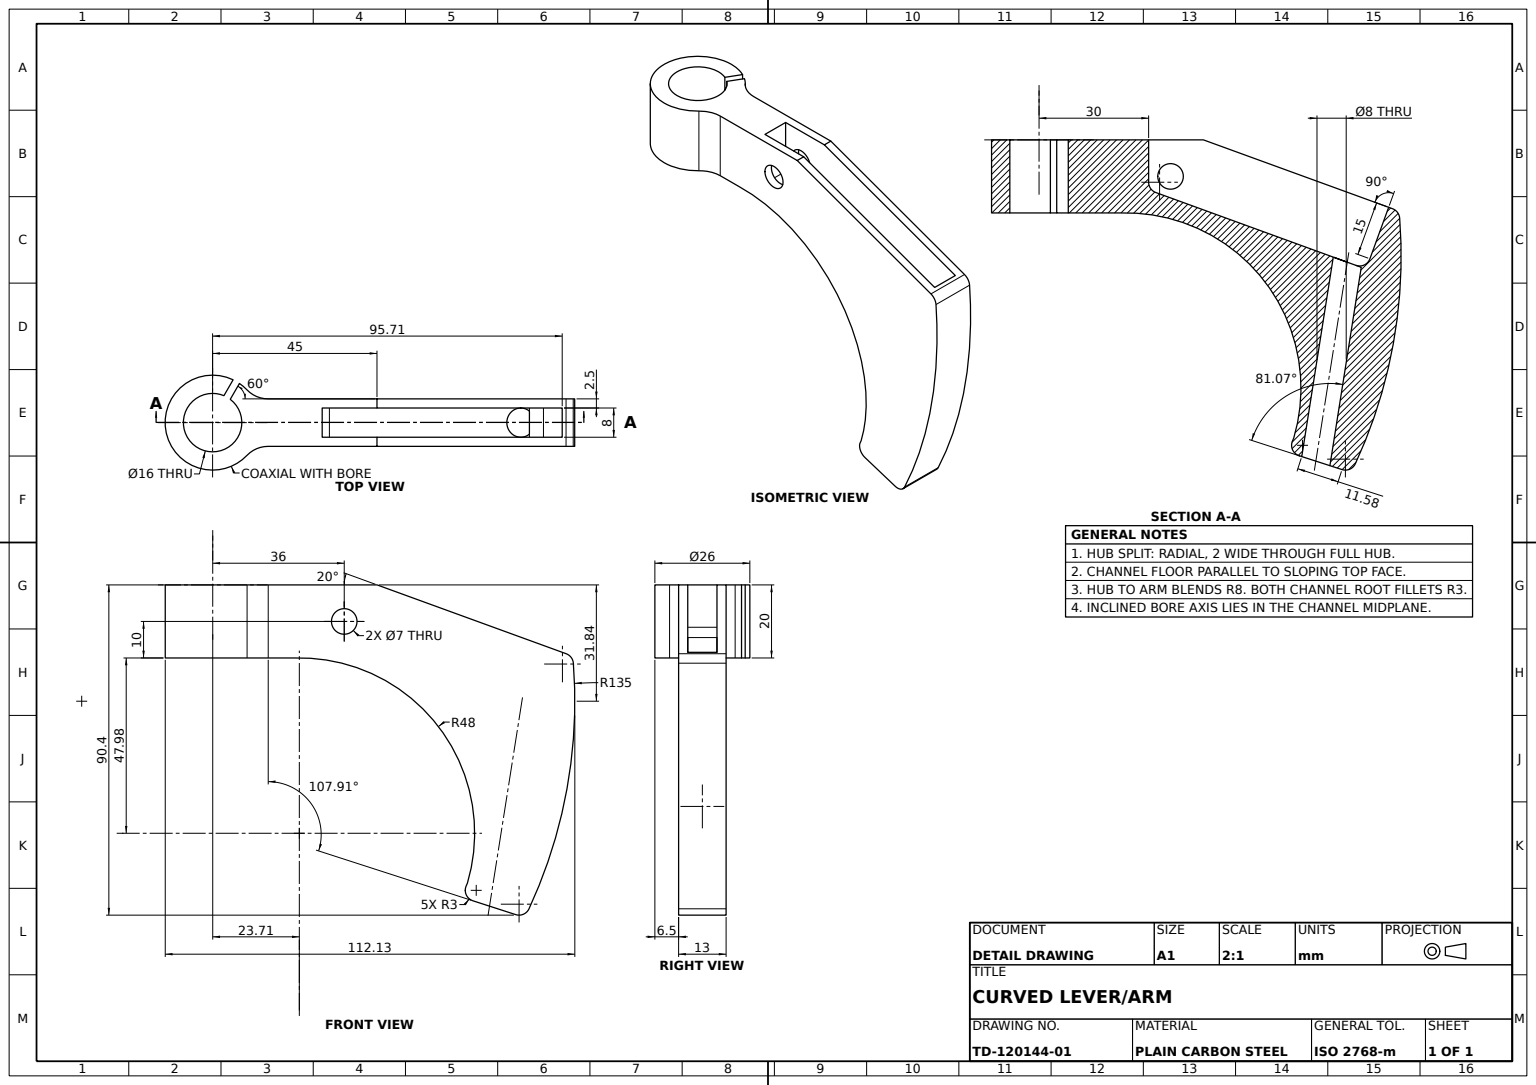
ISO-10303-21;
HEADER;
FILE_DESCRIPTION((''),'2;1');
FILE_NAME('','',(''),(''),'','','');
FILE_SCHEMA(('AUTOMOTIVE_DESIGN'));
ENDSEC;
DATA;
#1=APPLICATION_CONTEXT('');
#2=PRODUCT_CONTEXT('',#1,'mechanical');
#3=PRODUCT('','','',(#2));
#4=PRODUCT_DEFINITION_FORMATION('','',#3);
#5=PRODUCT_DEFINITION_CONTEXT('',#1,'design');
#6=PRODUCT_DEFINITION('','',#4,#5);
#7=PRODUCT_DEFINITION_SHAPE('','',#6);
#8=(LENGTH_UNIT()NAMED_UNIT(*)SI_UNIT(.MILLI.,.METRE.));
#9=(NAMED_UNIT(*)PLANE_ANGLE_UNIT()SI_UNIT($,.RADIAN.));
#10=(NAMED_UNIT(*)SI_UNIT($,.STERADIAN.)SOLID_ANGLE_UNIT());
#11=UNCERTAINTY_MEASURE_WITH_UNIT(LENGTH_MEASURE(1.E-05),#8,'distance_accuracy_value','');
#12=(GEOMETRIC_REPRESENTATION_CONTEXT(3)GLOBAL_UNCERTAINTY_ASSIGNED_CONTEXT((#11))GLOBAL_UNIT_ASSIGNED_CONTEXT((#8,#9,#10))REPRESENTATION_CONTEXT('',''));
#13=CARTESIAN_POINT('',(39.5,-10.,2.5));
#14=VERTEX_POINT('',#13);
#15=CARTESIAN_POINT('',(39.5,-10.,0.));
#16=VERTEX_POINT('',#15);
#17=CARTESIAN_POINT('',(39.5,-10.,13.));
#18=DIRECTION('',(0.,0.,-1.));
#19=VECTOR('',#18,1000.);
#20=LINE('',#17,#19);
#21=EDGE_CURVE('',#14,#16,#20,.T.);
#22=ORIENTED_EDGE('',*,*,#21,.F.);
#23=CARTESIAN_POINT('',(32.5,-10.,2.5));
#24=VERTEX_POINT('',#23);
#25=CARTESIAN_POINT('',(36.,-10.,2.5));
#26=DIRECTION('',(0.,0.,1.));
#27=DIRECTION('',(1.,0.,0.));
#28=AXIS2_PLACEMENT_3D('',#25,#26,#27);
#29=CIRCLE('',#28,3.5);
#30=EDGE_CURVE('',#14,#24,#29,.T.);
#31=ORIENTED_EDGE('',*,*,#30,.T.);
#32=CARTESIAN_POINT('',(32.5,-10.,0.));
#33=VERTEX_POINT('',#32);
#34=CARTESIAN_POINT('',(32.5,-10.,13.));
#35=LINE('',#34,#19);
#36=EDGE_CURVE('',#24,#33,#35,.T.);
#37=ORIENTED_EDGE('',*,*,#36,.T.);
#38=CARTESIAN_POINT('',(36.,-10.,0.));
#39=AXIS2_PLACEMENT_3D('',#38,#26,#27);
#40=CIRCLE('',#39,3.5);
#41=EDGE_CURVE('',#16,#33,#40,.T.);
#42=ORIENTED_EDGE('',*,*,#41,.F.);
#43=EDGE_LOOP('',(#22,#31,#37,#42));
#44=FACE_OUTER_BOUND('',#43,.T.);
#45=CARTESIAN_POINT('',(36.,-10.,13.));
#46=DIRECTION('',(-1.,0.,0.));
#47=AXIS2_PLACEMENT_3D('',#45,#18,#46);
#48=CYLINDRICAL_SURFACE('',#47,3.5);
#49=ADVANCED_FACE('',(#44),#48,.F.);
#50=CARTESIAN_POINT('',(30.,-11.595024,2.5));
#51=VERTEX_POINT('',#50);
#52=CARTESIAN_POINT('',(30.,-11.595024,10.5));
#53=VERTEX_POINT('',#52);
#54=VECTOR('',#26,1000.);
#55=LINE('',#50,#54);
#56=EDGE_CURVE('',#51,#53,#55,.T.);
#57=ORIENTED_EDGE('',*,*,#56,.T.);
#58=CARTESIAN_POINT('',(31.97394,-14.414102,10.5));
#59=VERTEX_POINT('',#58);
#60=CARTESIAN_POINT('',(33.,-11.595024,10.5));
#61=AXIS2_PLACEMENT_3D('',#60,#26,#46);
#62=CIRCLE('',#61,3.);
#63=EDGE_CURVE('',#53,#59,#62,.T.);
#64=ORIENTED_EDGE('',*,*,#63,.T.);
#65=CARTESIAN_POINT('',(31.97394,-14.414102,2.5));
#66=VERTEX_POINT('',#65);
#67=LINE('',#65,#54);
#68=EDGE_CURVE('',#66,#59,#67,.T.);
#69=ORIENTED_EDGE('',*,*,#68,.F.);
#70=CARTESIAN_POINT('',(33.,-11.595024,2.5));
#71=AXIS2_PLACEMENT_3D('',#70,#26,#46);
#72=CIRCLE('',#71,3.);
#73=EDGE_CURVE('',#51,#66,#72,.T.);
#74=ORIENTED_EDGE('',*,*,#73,.F.);
#75=EDGE_LOOP('',(#57,#64,#69,#74));
#76=FACE_OUTER_BOUND('',#75,.T.);
#77=AXIS2_PLACEMENT_3D('',#70,#26,#27);
#78=CYLINDRICAL_SURFACE('',#77,3.);
#79=ADVANCED_FACE('',(#76),#78,.F.);
#80=CARTESIAN_POINT('',(90.578301,-32.551811,10.5));
#81=VERTEX_POINT('',#80);
#82=CARTESIAN_POINT('',(95.708603,-18.456422,10.5));
#83=VERTEX_POINT('',#82);
#84=DIRECTION('',(0.342020143,0.939692621,0.));
#85=VECTOR('',#84,1000.);
#86=LINE('',#80,#85);
#87=EDGE_CURVE('',#81,#83,#86,.T.);
#88=ORIENTED_EDGE('',*,*,#87,.T.);
#89=CARTESIAN_POINT('',(95.708603,-18.456422,2.5));
#90=VERTEX_POINT('',#89);
#91=LINE('',#89,#54);
#92=EDGE_CURVE('',#90,#83,#91,.T.);
#93=ORIENTED_EDGE('',*,*,#92,.F.);
#94=CARTESIAN_POINT('',(90.578301,-32.551811,2.5));
#95=VERTEX_POINT('',#94);
#96=LINE('',#94,#85);
#97=EDGE_CURVE('',#95,#90,#96,.T.);
#98=ORIENTED_EDGE('',*,*,#97,.F.);
#99=LINE('',#94,#54);
#100=EDGE_CURVE('',#95,#81,#99,.T.);
#101=ORIENTED_EDGE('',*,*,#100,.T.);
#102=EDGE_LOOP('',(#88,#93,#98,#101));
#103=FACE_OUTER_BOUND('',#102,.T.);
#104=DIRECTION('',(0.939692621,-0.342020143,0.));
#105=AXIS2_PLACEMENT_3D('',#94,#104,#84);
#106=PLANE('',#105);
#107=ADVANCED_FACE('',(#103),#106,.F.);
#108=CARTESIAN_POINT('',(0.,-20.,-6.5));
#109=VERTEX_POINT('',#108);
#110=CARTESIAN_POINT('',(5.614715,-20.,-5.224972));
#111=VERTEX_POINT('',#110);
#112=CARTESIAN_POINT('',(0.,-20.,6.5));
#113=DIRECTION('',(0.,-1.,0.));
#114=AXIS2_PLACEMENT_3D('',#112,#113,#18);
#115=CIRCLE('',#114,13.);
#116=EDGE_CURVE('',#109,#111,#115,.T.);
#117=ORIENTED_EDGE('',*,*,#116,.F.);
#118=CARTESIAN_POINT('',(0.,0.,-6.5));
#119=VERTEX_POINT('',#118);
#120=VECTOR('',#113,1000.);
#121=LINE('',#108,#120);
#122=EDGE_CURVE('',#119,#109,#121,.T.);
#123=ORIENTED_EDGE('',*,*,#122,.F.);
#124=CARTESIAN_POINT('',(5.614715,0.,-5.224972));
#125=VERTEX_POINT('',#124);
#126=CARTESIAN_POINT('',(0.,0.,6.5));
#127=AXIS2_PLACEMENT_3D('',#126,#113,#18);
#128=CIRCLE('',#127,13.);
#129=EDGE_CURVE('',#119,#125,#128,.T.);
#130=ORIENTED_EDGE('',*,*,#129,.T.);
#131=LINE('',#110,#120);
#132=EDGE_CURVE('',#125,#111,#131,.T.);
#133=ORIENTED_EDGE('',*,*,#132,.T.);
#134=EDGE_LOOP('',(#117,#123,#130,#133));
#135=FACE_OUTER_BOUND('',#134,.T.);
#136=CYLINDRICAL_SURFACE('',#114,13.);
#137=ADVANCED_FACE('',(#135),#136,.T.);
#138=CARTESIAN_POINT('',(86.733162,-34.344829,9.653567));
#139=VERTEX_POINT('',#138);
#140=CARTESIAN_POINT('',(88.206809,-34.881192,6.5));
#141=VERTEX_POINT('',#140);
#142=CARTESIAN_POINT('',(87.680002,-34.68945,8.881841));
#143=CARTESIAN_POINT('',(88.206809,-34.881192,7.754486));
#144=(BOUNDED_CURVE()B_SPLINE_CURVE(3,(#138,#142,#143,#140),.UNSPECIFIED.,.F.,.T.)B_SPLINE_CURVE_WITH_KNOTS((4,4),(2.233402225,3.141592654),.UNSPECIFIED.)CURVE()GEOMETRIC_REPRESENTATION_ITEM()RATIONAL_B_SPLINE_CURVE((1.,0.932438853,0.932438853,1.))REPRESENTATION_ITEM(''));
#145=EDGE_CURVE('',#139,#141,#144,.T.);
#146=ORIENTED_EDGE('',*,*,#145,.T.);
#147=CARTESIAN_POINT('',(79.625923,-89.179734,6.5));
#148=VERTEX_POINT('',#147);
#149=CARTESIAN_POINT('',(78.754253,-94.695526,6.5));
#150=DIRECTION('',(0.156094482,0.987742129,0.));
#151=VECTOR('',#150,1000.);
#152=LINE('',#149,#151);
#153=EDGE_CURVE('',#148,#141,#152,.T.);
#154=ORIENTED_EDGE('',*,*,#153,.F.);
#155=CARTESIAN_POINT('',(71.920122,-86.689858,6.5));
#156=VERTEX_POINT('',#155);
#157=CARTESIAN_POINT('',(71.920122,-86.689858,14.5));
#158=CARTESIAN_POINT('',(79.625923,-89.179734,14.5));
#159=(BOUNDED_CURVE()B_SPLINE_CURVE(3,(#155,#157,#158,#147),.UNSPECIFIED.,.F.,.T.)B_SPLINE_CURVE_WITH_KNOTS((4,4),(0.,3.141592654),.UNSPECIFIED.)CURVE()GEOMETRIC_REPRESENTATION_ITEM()RATIONAL_B_SPLINE_CURVE((1.,0.333333333,0.333333333,1.))REPRESENTATION_ITEM(''));
#160=EDGE_CURVE('',#156,#148,#159,.T.);
#161=ORIENTED_EDGE('',*,*,#160,.F.);
#162=CARTESIAN_POINT('',(80.548052,-32.093633,6.5));
#163=VERTEX_POINT('',#162);
#164=CARTESIAN_POINT('',(70.852316,-93.44677,6.5));
#165=LINE('',#164,#151);
#166=EDGE_CURVE('',#156,#163,#165,.T.);
#167=ORIENTED_EDGE('',*,*,#166,.T.);
#168=CARTESIAN_POINT('',(84.37743,-33.487412,10.5));
#169=VERTEX_POINT('',#168);
#170=CARTESIAN_POINT('',(80.548052,-32.093633,8.843146));
#171=CARTESIAN_POINT('',(82.134232,-32.670955,10.5));
#172=(BOUNDED_CURVE()B_SPLINE_CURVE(3,(#162,#170,#171,#168),.UNSPECIFIED.,.F.,.T.)B_SPLINE_CURVE_WITH_KNOTS((4,4),(0.,1.570796327),.UNSPECIFIED.)CURVE()GEOMETRIC_REPRESENTATION_ITEM()RATIONAL_B_SPLINE_CURVE((1.,0.804737854,0.804737854,1.))REPRESENTATION_ITEM(''));
#173=EDGE_CURVE('',#163,#169,#172,.T.);
#174=ORIENTED_EDGE('',*,*,#173,.T.);
#175=CARTESIAN_POINT('',(85.23907,-33.801024,10.5));
#176=CARTESIAN_POINT('',(86.053853,-34.09758,10.207242));
#177=(BOUNDED_CURVE()B_SPLINE_CURVE(3,(#168,#175,#176,#138),.UNSPECIFIED.,.F.,.T.)B_SPLINE_CURVE_WITH_KNOTS((4,4),(1.570796327,2.233402225),.UNSPECIFIED.)CURVE()GEOMETRIC_REPRESENTATION_ITEM()RATIONAL_B_SPLINE_CURVE((1.,0.963746219,0.963746219,1.))REPRESENTATION_ITEM(''));
#178=EDGE_CURVE('',#169,#139,#177,.T.);
#179=ORIENTED_EDGE('',*,*,#178,.T.);
#180=EDGE_LOOP('',(#146,#154,#161,#167,#174,#179));
#181=FACE_OUTER_BOUND('',#180,.T.);
#182=CARTESIAN_POINT('',(74.803285,-94.071148,6.5));
#183=DIRECTION('',(-0.987742129,0.156094482,0.));
#184=AXIS2_PLACEMENT_3D('',#182,#150,#183);
#185=CYLINDRICAL_SURFACE('',#184,4.);
#186=ADVANCED_FACE('',(#181),#185,.F.);
#187=CARTESIAN_POINT('',(4.834652,0.,0.126136));
#188=VERTEX_POINT('',#187);
#189=CARTESIAN_POINT('',(0.,0.,14.5));
#190=VERTEX_POINT('',#189);
#191=CIRCLE('',#127,8.);
#192=EDGE_CURVE('',#188,#190,#191,.T.);
#193=ORIENTED_EDGE('',*,*,#192,.F.);
#194=CARTESIAN_POINT('',(4.834652,-20.,0.126136));
#195=VERTEX_POINT('',#194);
#196=LINE('',#194,#120);
#197=EDGE_CURVE('',#188,#195,#196,.T.);
#198=ORIENTED_EDGE('',*,*,#197,.T.);
#199=CARTESIAN_POINT('',(0.,-20.,14.5));
#200=VERTEX_POINT('',#199);
#201=CIRCLE('',#114,8.);
#202=EDGE_CURVE('',#195,#200,#201,.T.);
#203=ORIENTED_EDGE('',*,*,#202,.T.);
#204=LINE('',#199,#120);
#205=EDGE_CURVE('',#190,#200,#204,.T.);
#206=ORIENTED_EDGE('',*,*,#205,.F.);
#207=EDGE_LOOP('',(#193,#198,#203,#206));
#208=FACE_OUTER_BOUND('',#207,.T.);
#209=CYLINDRICAL_SURFACE('',#114,8.);
#210=ADVANCED_FACE('',(#208),#209,.F.);
#211=CARTESIAN_POINT('',(30.,0.,10.5));
#212=VERTEX_POINT('',#211);
#213=LINE('',#211,#120);
#214=EDGE_CURVE('',#212,#53,#213,.T.);
#215=ORIENTED_EDGE('',*,*,#214,.T.);
#216=ORIENTED_EDGE('',*,*,#56,.F.);
#217=CARTESIAN_POINT('',(30.,0.,2.5));
#218=VERTEX_POINT('',#217);
#219=LINE('',#217,#120);
#220=EDGE_CURVE('',#218,#51,#219,.T.);
#221=ORIENTED_EDGE('',*,*,#220,.F.);
#222=LINE('',#217,#54);
#223=EDGE_CURVE('',#218,#212,#222,.T.);
#224=ORIENTED_EDGE('',*,*,#223,.T.);
#225=EDGE_LOOP('',(#215,#216,#221,#224));
#226=FACE_OUTER_BOUND('',#225,.T.);
#227=AXIS2_PLACEMENT_3D('',#217,#46,#113);
#228=PLANE('',#227);
#229=ADVANCED_FACE('',(#226),#228,.F.);
#230=CARTESIAN_POINT('',(3.102602,-20.,-0.873864));
#231=VERTEX_POINT('',#230);
#232=CARTESIAN_POINT('',(3.102602,0.,-0.873864));
#233=VERTEX_POINT('',#232);
#234=DIRECTION('',(0.,1.,0.));
#235=VECTOR('',#234,1000.);
#236=LINE('',#230,#235);
#237=EDGE_CURVE('',#231,#233,#236,.T.);
#238=ORIENTED_EDGE('',*,*,#237,.F.);
#239=CARTESIAN_POINT('',(-3.680608,-20.,10.875));
#240=DIRECTION('',(-0.5,0.,0.866025404));
#241=VECTOR('',#240,1000.);
#242=LINE('',#239,#241);
#243=EDGE_CURVE('',#111,#231,#242,.T.);
#244=ORIENTED_EDGE('',*,*,#243,.F.);
#245=ORIENTED_EDGE('',*,*,#132,.F.);
#246=CARTESIAN_POINT('',(2.598076,0.,0.));
#247=LINE('',#246,#241);
#248=EDGE_CURVE('',#125,#233,#247,.T.);
#249=ORIENTED_EDGE('',*,*,#248,.T.);
#250=EDGE_LOOP('',(#238,#244,#245,#249));
#251=FACE_OUTER_BOUND('',#250,.T.);
#252=CARTESIAN_POINT('',(2.598076,-53.,0.));
#253=DIRECTION('',(-0.866025404,0.,-0.5));
#254=AXIS2_PLACEMENT_3D('',#252,#253,#240);
#255=PLANE('',#254);
#256=ADVANCED_FACE('',(#251),#255,.F.);
#257=CARTESIAN_POINT('',(69.13471,-83.606475,13.));
#258=VERTEX_POINT('',#257);
#259=CARTESIAN_POINT('',(69.13471,-83.606475,0.));
#260=VERTEX_POINT('',#259);
#261=LINE('',#257,#19);
#262=EDGE_CURVE('',#258,#260,#261,.T.);
#263=ORIENTED_EDGE('',*,*,#262,.F.);
#264=CARTESIAN_POINT('',(69.382465,-82.41268,13.));
#265=VERTEX_POINT('',#264);
#266=CARTESIAN_POINT('',(72.13471,-83.606475,13.));
#267=AXIS2_PLACEMENT_3D('',#266,#26,#46);
#268=CIRCLE('',#267,3.);
#269=EDGE_CURVE('',#265,#258,#268,.T.);
#270=ORIENTED_EDGE('',*,*,#269,.F.);
#271=CARTESIAN_POINT('',(69.382465,-82.41268,0.));
#272=VERTEX_POINT('',#271);
#273=LINE('',#264,#54);
#274=EDGE_CURVE('',#272,#265,#273,.T.);
#275=ORIENTED_EDGE('',*,*,#274,.F.);
#276=CARTESIAN_POINT('',(72.13471,-83.606475,0.));
#277=AXIS2_PLACEMENT_3D('',#276,#18,#46);
#278=CIRCLE('',#277,3.);
#279=EDGE_CURVE('',#260,#272,#278,.T.);
#280=ORIENTED_EDGE('',*,*,#279,.F.);
#281=EDGE_LOOP('',(#263,#270,#275,#280));
#282=FACE_OUTER_BOUND('',#281,.T.);
#283=AXIS2_PLACEMENT_3D('',#266,#18,#46);
#284=CYLINDRICAL_SURFACE('',#283,3.);
#285=ADVANCED_FACE('',(#282),#284,.T.);
#286=CARTESIAN_POINT('',(86.586333,-88.659483,13.));
#287=VERTEX_POINT('',#286);
#288=CARTESIAN_POINT('',(86.586333,-88.659483,0.));
#289=VERTEX_POINT('',#288);
#290=LINE('',#286,#19);
#291=EDGE_CURVE('',#287,#289,#290,.T.);
#292=ORIENTED_EDGE('',*,*,#291,.F.);
#293=CARTESIAN_POINT('',(82.942635,-90.25142,13.));
#294=VERTEX_POINT('',#293);
#295=CARTESIAN_POINT('',(83.865031,-87.396742,13.));
#296=AXIS2_PLACEMENT_3D('',#295,#26,#46);
#297=CIRCLE('',#296,3.);
#298=EDGE_CURVE('',#294,#287,#297,.T.);
#299=ORIENTED_EDGE('',*,*,#298,.F.);
#300=CARTESIAN_POINT('',(82.942635,-90.25142,0.));
#301=VERTEX_POINT('',#300);
#302=LINE('',#293,#54);
#303=EDGE_CURVE('',#301,#294,#302,.T.);
#304=ORIENTED_EDGE('',*,*,#303,.F.);
#305=CARTESIAN_POINT('',(83.865031,-87.396742,0.));
#306=AXIS2_PLACEMENT_3D('',#305,#18,#46);
#307=CIRCLE('',#306,3.);
#308=EDGE_CURVE('',#289,#301,#307,.T.);
#309=ORIENTED_EDGE('',*,*,#308,.F.);
#310=EDGE_LOOP('',(#292,#299,#304,#309));
#311=FACE_OUTER_BOUND('',#310,.T.);
#312=AXIS2_PLACEMENT_3D('',#295,#18,#46);
#313=CYLINDRICAL_SURFACE('',#312,3.);
#314=ADVANCED_FACE('',(#311),#313,.T.);
#315=CARTESIAN_POINT('',(69.730755,-81.609712,13.));
#316=VERTEX_POINT('',#315);
#317=CARTESIAN_POINT('',(69.730755,-81.609712,0.));
#318=VERTEX_POINT('',#317);
#319=LINE('',#315,#19);
#320=EDGE_CURVE('',#316,#318,#319,.T.);
#321=ORIENTED_EDGE('',*,*,#320,.F.);
#322=CARTESIAN_POINT('',(22.459983,-20.,13.));
#323=VERTEX_POINT('',#322);
#324=CARTESIAN_POINT('',(23.705375,-67.983841,13.));
#325=AXIS2_PLACEMENT_3D('',#324,#18,#46);
#326=CIRCLE('',#325,48.);
#327=EDGE_CURVE('',#323,#316,#326,.T.);
#328=ORIENTED_EDGE('',*,*,#327,.F.);
#329=CARTESIAN_POINT('',(22.459983,-20.,0.));
#330=VERTEX_POINT('',#329);
#331=LINE('',#322,#19);
#332=EDGE_CURVE('',#323,#330,#331,.T.);
#333=ORIENTED_EDGE('',*,*,#332,.T.);
#334=CARTESIAN_POINT('',(23.705375,-67.983841,0.));
#335=AXIS2_PLACEMENT_3D('',#334,#18,#46);
#336=CIRCLE('',#335,48.);
#337=EDGE_CURVE('',#330,#318,#336,.T.);
#338=ORIENTED_EDGE('',*,*,#337,.T.);
#339=EDGE_LOOP('',(#321,#328,#333,#338));
#340=FACE_OUTER_BOUND('',#339,.T.);
#341=CYLINDRICAL_SURFACE('',#325,48.);
#342=ADVANCED_FACE('',(#340),#341,.F.);
#343=ORIENTED_EDGE('',*,*,#192,.T.);
#344=CARTESIAN_POINT('',(0.,0.,-1.5));
#345=VERTEX_POINT('',#344);
#346=EDGE_CURVE('',#190,#345,#191,.T.);
#347=ORIENTED_EDGE('',*,*,#346,.T.);
#348=EDGE_CURVE('',#345,#233,#191,.T.);
#349=ORIENTED_EDGE('',*,*,#348,.T.);
#350=ORIENTED_EDGE('',*,*,#248,.F.);
#351=ORIENTED_EDGE('',*,*,#129,.F.);
#352=CARTESIAN_POINT('',(0.,0.,19.5));
#353=VERTEX_POINT('',#352);
#354=EDGE_CURVE('',#353,#119,#128,.T.);
#355=ORIENTED_EDGE('',*,*,#354,.F.);
#356=CARTESIAN_POINT('',(9.403617,0.,15.47619));
#357=VERTEX_POINT('',#356);
#358=EDGE_CURVE('',#357,#353,#128,.T.);
#359=ORIENTED_EDGE('',*,*,#358,.F.);
#360=CARTESIAN_POINT('',(15.190458,0.,13.));
#361=VERTEX_POINT('',#360);
#362=CARTESIAN_POINT('',(15.190458,0.,21.));
#363=AXIS2_PLACEMENT_3D('',#362,#113,#18);
#364=CIRCLE('',#363,8.);
#365=EDGE_CURVE('',#357,#361,#364,.T.);
#366=ORIENTED_EDGE('',*,*,#365,.T.);
#367=CARTESIAN_POINT('',(45.,0.,13.));
#368=VERTEX_POINT('',#367);
#369=CARTESIAN_POINT('',(0.,0.,13.));
#370=VECTOR('',#46,1000.);
#371=LINE('',#369,#370);
#372=EDGE_CURVE('',#368,#361,#371,.T.);
#373=ORIENTED_EDGE('',*,*,#372,.F.);
#374=CARTESIAN_POINT('',(45.,0.,10.5));
#375=VERTEX_POINT('',#374);
#376=LINE('',#367,#19);
#377=EDGE_CURVE('',#368,#375,#376,.T.);
#378=ORIENTED_EDGE('',*,*,#377,.T.);
#379=LINE('',#211,#370);
#380=EDGE_CURVE('',#375,#212,#379,.T.);
#381=ORIENTED_EDGE('',*,*,#380,.T.);
#382=ORIENTED_EDGE('',*,*,#223,.F.);
#383=CARTESIAN_POINT('',(45.,0.,2.5));
#384=VERTEX_POINT('',#383);
#385=LINE('',#217,#370);
#386=EDGE_CURVE('',#384,#218,#385,.T.);
#387=ORIENTED_EDGE('',*,*,#386,.F.);
#388=CARTESIAN_POINT('',(45.,0.,0.));
#389=VERTEX_POINT('',#388);
#390=EDGE_CURVE('',#384,#389,#376,.T.);
#391=ORIENTED_EDGE('',*,*,#390,.T.);
#392=CARTESIAN_POINT('',(15.190458,0.,0.));
#393=VERTEX_POINT('',#392);
#394=CARTESIAN_POINT('',(0.,0.,0.));
#395=LINE('',#394,#370);
#396=EDGE_CURVE('',#389,#393,#395,.T.);
#397=ORIENTED_EDGE('',*,*,#396,.T.);
#398=CARTESIAN_POINT('',(9.403617,0.,-2.47619));
#399=VERTEX_POINT('',#398);
#400=CARTESIAN_POINT('',(15.190458,0.,-8.));
#401=AXIS2_PLACEMENT_3D('',#400,#113,#18);
#402=CIRCLE('',#401,8.);
#403=EDGE_CURVE('',#393,#399,#402,.T.);
#404=ORIENTED_EDGE('',*,*,#403,.T.);
#405=CARTESIAN_POINT('',(7.346766,0.,-4.224972));
#406=VERTEX_POINT('',#405);
#407=EDGE_CURVE('',#406,#399,#128,.T.);
#408=ORIENTED_EDGE('',*,*,#407,.F.);
#409=CARTESIAN_POINT('',(4.330127,0.,1.));
#410=DIRECTION('',(0.5,0.,-0.866025404));
#411=VECTOR('',#410,1000.);
#412=LINE('',#409,#411);
#413=EDGE_CURVE('',#188,#406,#412,.T.);
#414=ORIENTED_EDGE('',*,*,#413,.F.);
#415=EDGE_LOOP('',(#343,#347,#349,#350,#351,#355,#359,#366,#373,#378,#381,#382,#387,#391,#397,#404,#408,#414));
#416=FACE_OUTER_BOUND('',#415,.T.);
#417=AXIS2_PLACEMENT_3D('',#369,#113,#18);
#418=PLANE('',#417);
#419=ADVANCED_FACE('',(#416),#418,.F.);
#420=CARTESIAN_POINT('',(9.403617,-20.,-2.47619));
#421=VERTEX_POINT('',#420);
#422=CARTESIAN_POINT('',(15.190458,-20.,0.));
#423=VERTEX_POINT('',#422);
#424=CARTESIAN_POINT('',(15.190458,-20.,-8.));
#425=AXIS2_PLACEMENT_3D('',#424,#234,#46);
#426=CIRCLE('',#425,8.);
#427=EDGE_CURVE('',#421,#423,#426,.T.);
#428=ORIENTED_EDGE('',*,*,#427,.F.);
#429=LINE('',#420,#120);
#430=EDGE_CURVE('',#399,#421,#429,.T.);
#431=ORIENTED_EDGE('',*,*,#430,.F.);
#432=ORIENTED_EDGE('',*,*,#403,.F.);
#433=CARTESIAN_POINT('',(15.190458,-67.983841,0.));
#434=LINE('',#433,#235);
#435=EDGE_CURVE('',#423,#393,#434,.T.);
#436=ORIENTED_EDGE('',*,*,#435,.F.);
#437=EDGE_LOOP('',(#428,#431,#432,#436));
#438=FACE_OUTER_BOUND('',#437,.T.);
#439=AXIS2_PLACEMENT_3D('',#424,#113,#18);
#440=CYLINDRICAL_SURFACE('',#439,8.);
#441=ADVANCED_FACE('',(#438),#440,.F.);
#442=CARTESIAN_POINT('',(96.760847,-18.839407,13.));
#443=VERTEX_POINT('',#442);
#444=CARTESIAN_POINT('',(96.760847,-18.839407,0.));
#445=VERTEX_POINT('',#444);
#446=LINE('',#442,#19);
#447=EDGE_CURVE('',#443,#445,#446,.T.);
#448=ORIENTED_EDGE('',*,*,#447,.F.);
#449=CARTESIAN_POINT('',(98.725855,-21.427175,13.));
#450=VERTEX_POINT('',#449);
#451=CARTESIAN_POINT('',(95.734786,-21.658485,13.));
#452=AXIS2_PLACEMENT_3D('',#451,#26,#46);
#453=CIRCLE('',#452,3.);
#454=EDGE_CURVE('',#450,#443,#453,.T.);
#455=ORIENTED_EDGE('',*,*,#454,.F.);
#456=CARTESIAN_POINT('',(98.725855,-21.427175,0.));
#457=VERTEX_POINT('',#456);
#458=LINE('',#449,#19);
#459=EDGE_CURVE('',#450,#457,#458,.T.);
#460=ORIENTED_EDGE('',*,*,#459,.T.);
#461=CARTESIAN_POINT('',(95.734786,-21.658485,0.));
#462=AXIS2_PLACEMENT_3D('',#461,#26,#46);
#463=CIRCLE('',#462,3.);
#464=EDGE_CURVE('',#457,#445,#463,.T.);
#465=ORIENTED_EDGE('',*,*,#464,.T.);
#466=EDGE_LOOP('',(#448,#455,#460,#465));
#467=FACE_OUTER_BOUND('',#466,.T.);
#468=AXIS2_PLACEMENT_3D('',#451,#18,#46);
#469=CYLINDRICAL_SURFACE('',#468,3.);
#470=ADVANCED_FACE('',(#467),#469,.T.);
#471=CARTESIAN_POINT('',(71.212315,-86.461153,13.));
#472=VERTEX_POINT('',#471);
#473=CARTESIAN_POINT('',(68.067222,-85.44492,13.));
#474=DIRECTION('',(0.95155936,-0.307465094,0.));
#475=VECTOR('',#474,1000.);
#476=LINE('',#473,#475);
#477=EDGE_CURVE('',#472,#294,#476,.T.);
#478=ORIENTED_EDGE('',*,*,#477,.F.);
#479=CARTESIAN_POINT('',(71.212315,-86.461153,0.));
#480=VERTEX_POINT('',#479);
#481=LINE('',#471,#19);
#482=EDGE_CURVE('',#472,#480,#481,.T.);
#483=ORIENTED_EDGE('',*,*,#482,.T.);
#484=CARTESIAN_POINT('',(68.067222,-85.44492,0.));
#485=LINE('',#484,#475);
#486=EDGE_CURVE('',#480,#301,#485,.T.);
#487=ORIENTED_EDGE('',*,*,#486,.T.);
#488=ORIENTED_EDGE('',*,*,#303,.T.);
#489=EDGE_LOOP('',(#478,#483,#487,#488));
#490=FACE_OUTER_BOUND('',#489,.T.);
#491=ORIENTED_EDGE('',*,*,#160,.T.);
#492=CARTESIAN_POINT('',(79.625923,-89.179734,-1.5));
#493=CARTESIAN_POINT('',(71.920122,-86.689858,-1.5));
#494=(BOUNDED_CURVE()B_SPLINE_CURVE(3,(#147,#492,#493,#155),.UNSPECIFIED.,.F.,.F.)B_SPLINE_CURVE_WITH_KNOTS((4,4),(3.141592654,6.283185307),.UNSPECIFIED.)CURVE()GEOMETRIC_REPRESENTATION_ITEM()RATIONAL_B_SPLINE_CURVE((1.,0.333333333,0.333333333,1.))REPRESENTATION_ITEM(''));
#495=EDGE_CURVE('',#148,#156,#494,.T.);
#496=ORIENTED_EDGE('',*,*,#495,.T.);
#497=EDGE_LOOP('',(#491,#496));
#498=FACE_BOUND('',#497,.T.);
#499=DIRECTION('',(0.307465094,0.95155936,0.));
#500=DIRECTION('',(-0.95155936,0.307465094,0.));
#501=AXIS2_PLACEMENT_3D('',#473,#499,#500);
#502=PLANE('',#501);
#503=ADVANCED_FACE('',(#490,#498),#502,.F.);
#504=ORIENTED_EDGE('',*,*,#68,.T.);
#505=CARTESIAN_POINT('',(86.733162,-34.344829,10.5));
#506=VECTOR('',#104,1000.);
#507=LINE('',#505,#506);
#508=EDGE_CURVE('',#59,#169,#507,.T.);
#509=ORIENTED_EDGE('',*,*,#508,.T.);
#510=ORIENTED_EDGE('',*,*,#173,.F.);
#511=CARTESIAN_POINT('',(84.37743,-33.487412,2.5));
#512=VERTEX_POINT('',#511);
#513=CARTESIAN_POINT('',(82.134232,-32.670955,2.5));
#514=CARTESIAN_POINT('',(80.548052,-32.093633,4.156854));
#515=(BOUNDED_CURVE()B_SPLINE_CURVE(3,(#511,#513,#514,#162),.UNSPECIFIED.,.F.,.T.)B_SPLINE_CURVE_WITH_KNOTS((4,4),(4.71238898,6.283185307),.UNSPECIFIED.)CURVE()GEOMETRIC_REPRESENTATION_ITEM()RATIONAL_B_SPLINE_CURVE((1.,0.804737854,0.804737854,1.))REPRESENTATION_ITEM(''));
#516=EDGE_CURVE('',#512,#163,#515,.T.);
#517=ORIENTED_EDGE('',*,*,#516,.F.);
#518=CARTESIAN_POINT('',(86.733162,-34.344829,2.5));
#519=LINE('',#518,#506);
#520=EDGE_CURVE('',#66,#512,#519,.T.);
#521=ORIENTED_EDGE('',*,*,#520,.F.);
#522=EDGE_LOOP('',(#504,#509,#510,#517,#521));
#523=FACE_OUTER_BOUND('',#522,.T.);
#524=DIRECTION('',(-0.342020143,-0.939692621,0.));
#525=AXIS2_PLACEMENT_3D('',#518,#524,#104);
#526=PLANE('',#525);
#527=ADVANCED_FACE('',(#523),#526,.F.);
#528=CARTESIAN_POINT('',(7.346766,-20.,-4.224972));
#529=VERTEX_POINT('',#528);
#530=CARTESIAN_POINT('',(-1.948557,-20.,11.875));
#531=LINE('',#530,#411);
#532=EDGE_CURVE('',#195,#529,#531,.T.);
#533=ORIENTED_EDGE('',*,*,#532,.F.);
#534=ORIENTED_EDGE('',*,*,#197,.F.);
#535=ORIENTED_EDGE('',*,*,#413,.T.);
#536=LINE('',#528,#235);
#537=EDGE_CURVE('',#529,#406,#536,.T.);
#538=ORIENTED_EDGE('',*,*,#537,.F.);
#539=EDGE_LOOP('',(#533,#534,#535,#538));
#540=FACE_OUTER_BOUND('',#539,.T.);
#541=CARTESIAN_POINT('',(4.330127,-53.,1.));
#542=DIRECTION('',(0.866025404,0.,0.5));
#543=AXIS2_PLACEMENT_3D('',#541,#542,#410);
#544=PLANE('',#543);
#545=ADVANCED_FACE('',(#540),#544,.F.);
#546=ORIENTED_EDGE('',*,*,#92,.T.);
#547=DIRECTION('',(-0.939692621,0.342020143,0.));
#548=VECTOR('',#547,1000.);
#549=LINE('',#82,#548);
#550=EDGE_CURVE('',#83,#375,#549,.T.);
#551=ORIENTED_EDGE('',*,*,#550,.T.);
#552=ORIENTED_EDGE('',*,*,#377,.F.);
#553=LINE('',#367,#548);
#554=EDGE_CURVE('',#443,#368,#553,.T.);
#555=ORIENTED_EDGE('',*,*,#554,.F.);
#556=ORIENTED_EDGE('',*,*,#447,.T.);
#557=LINE('',#388,#548);
#558=EDGE_CURVE('',#445,#389,#557,.T.);
#559=ORIENTED_EDGE('',*,*,#558,.T.);
#560=ORIENTED_EDGE('',*,*,#390,.F.);
#561=LINE('',#89,#548);
#562=EDGE_CURVE('',#90,#384,#561,.T.);
#563=ORIENTED_EDGE('',*,*,#562,.F.);
#564=EDGE_LOOP('',(#546,#551,#552,#555,#556,#559,#560,#563));
#565=FACE_OUTER_BOUND('',#564,.T.);
#566=AXIS2_PLACEMENT_3D('',#367,#524,#104);
#567=PLANE('',#566);
#568=ADVANCED_FACE('',(#565),#567,.F.);
#569=CARTESIAN_POINT('',(0.,-20.,19.5));
#570=VERTEX_POINT('',#569);
#571=LINE('',#569,#120);
#572=EDGE_CURVE('',#353,#570,#571,.T.);
#573=ORIENTED_EDGE('',*,*,#572,.T.);
#574=CARTESIAN_POINT('',(9.403617,-20.,15.47619));
#575=VERTEX_POINT('',#574);
#576=EDGE_CURVE('',#575,#570,#115,.T.);
#577=ORIENTED_EDGE('',*,*,#576,.F.);
#578=LINE('',#574,#235);
#579=EDGE_CURVE('',#575,#357,#578,.T.);
#580=ORIENTED_EDGE('',*,*,#579,.T.);
#581=ORIENTED_EDGE('',*,*,#358,.T.);
#582=EDGE_LOOP('',(#573,#577,#580,#581));
#583=FACE_OUTER_BOUND('',#582,.T.);
#584=ADVANCED_FACE('',(#583),#136,.T.);
#585=ORIENTED_EDGE('',*,*,#346,.F.);
#586=ORIENTED_EDGE('',*,*,#205,.T.);
#587=CARTESIAN_POINT('',(0.,-20.,-1.5));
#588=VERTEX_POINT('',#587);
#589=EDGE_CURVE('',#200,#588,#201,.T.);
#590=ORIENTED_EDGE('',*,*,#589,.T.);
#591=LINE('',#587,#120);
#592=EDGE_CURVE('',#345,#588,#591,.T.);
#593=ORIENTED_EDGE('',*,*,#592,.F.);
#594=EDGE_LOOP('',(#585,#586,#590,#593));
#595=FACE_OUTER_BOUND('',#594,.T.);
#596=ADVANCED_FACE('',(#595),#209,.F.);
#597=CARTESIAN_POINT('',(39.5,-10.,10.5));
#598=VERTEX_POINT('',#597);
#599=CARTESIAN_POINT('',(32.5,-10.,10.5));
#600=VERTEX_POINT('',#599);
#601=CARTESIAN_POINT('',(36.,-10.,10.5));
#602=AXIS2_PLACEMENT_3D('',#601,#26,#27);
#603=CIRCLE('',#602,3.5);
#604=EDGE_CURVE('',#598,#600,#603,.T.);
#605=ORIENTED_EDGE('',*,*,#604,.F.);
#606=VERTEX_POINT('',#17);
#607=EDGE_CURVE('',#606,#598,#20,.T.);
#608=ORIENTED_EDGE('',*,*,#607,.F.);
#609=VERTEX_POINT('',#34);
#610=AXIS2_PLACEMENT_3D('',#45,#26,#27);
#611=CIRCLE('',#610,3.5);
#612=EDGE_CURVE('',#606,#609,#611,.T.);
#613=ORIENTED_EDGE('',*,*,#612,.T.);
#614=EDGE_CURVE('',#609,#600,#35,.T.);
#615=ORIENTED_EDGE('',*,*,#614,.T.);
#616=EDGE_LOOP('',(#605,#608,#613,#615));
#617=FACE_OUTER_BOUND('',#616,.T.);
#618=ADVANCED_FACE('',(#617),#48,.F.);
#619=EDGE_CURVE('',#529,#421,#115,.T.);
#620=ORIENTED_EDGE('',*,*,#619,.F.);
#621=ORIENTED_EDGE('',*,*,#537,.T.);
#622=ORIENTED_EDGE('',*,*,#407,.T.);
#623=ORIENTED_EDGE('',*,*,#430,.T.);
#624=EDGE_LOOP('',(#620,#621,#622,#623));
#625=FACE_OUTER_BOUND('',#624,.T.);
#626=ADVANCED_FACE('',(#625),#136,.T.);
#627=ORIENTED_EDGE('',*,*,#202,.F.);
#628=ORIENTED_EDGE('',*,*,#532,.T.);
#629=ORIENTED_EDGE('',*,*,#619,.T.);
#630=ORIENTED_EDGE('',*,*,#427,.T.);
#631=CARTESIAN_POINT('',(0.,-20.,0.));
#632=VECTOR('',#27,1000.);
#633=LINE('',#631,#632);
#634=EDGE_CURVE('',#423,#330,#633,.T.);
#635=ORIENTED_EDGE('',*,*,#634,.T.);
#636=ORIENTED_EDGE('',*,*,#332,.F.);
#637=CARTESIAN_POINT('',(15.190458,-20.,13.));
#638=VERTEX_POINT('',#637);
#639=CARTESIAN_POINT('',(0.,-20.,13.));
#640=LINE('',#639,#632);
#641=EDGE_CURVE('',#638,#323,#640,.T.);
#642=ORIENTED_EDGE('',*,*,#641,.F.);
#643=CARTESIAN_POINT('',(15.190458,-20.,21.));
#644=AXIS2_PLACEMENT_3D('',#643,#234,#46);
#645=CIRCLE('',#644,8.);
#646=EDGE_CURVE('',#638,#575,#645,.T.);
#647=ORIENTED_EDGE('',*,*,#646,.T.);
#648=ORIENTED_EDGE('',*,*,#576,.T.);
#649=EDGE_CURVE('',#570,#109,#115,.T.);
#650=ORIENTED_EDGE('',*,*,#649,.T.);
#651=ORIENTED_EDGE('',*,*,#116,.T.);
#652=ORIENTED_EDGE('',*,*,#243,.T.);
#653=EDGE_CURVE('',#588,#231,#201,.T.);
#654=ORIENTED_EDGE('',*,*,#653,.F.);
#655=ORIENTED_EDGE('',*,*,#589,.F.);
#656=EDGE_LOOP('',(#627,#628,#629,#630,#635,#636,#642,#647,#648,#650,#651,#652,#654,#655));
#657=FACE_OUTER_BOUND('',#656,.T.);
#658=AXIS2_PLACEMENT_3D('',#639,#234,#46);
#659=PLANE('',#658);
#660=ADVANCED_FACE('',(#657),#659,.F.);
#661=ORIENTED_EDGE('',*,*,#435,.T.);
#662=ORIENTED_EDGE('',*,*,#396,.F.);
#663=ORIENTED_EDGE('',*,*,#558,.F.);
#664=ORIENTED_EDGE('',*,*,#464,.F.);
#665=CARTESIAN_POINT('',(-35.872263,-31.83614,0.));
#666=AXIS2_PLACEMENT_3D('',#665,#26,#46);
#667=CIRCLE('',#666,135.);
#668=EDGE_CURVE('',#289,#457,#667,.T.);
#669=ORIENTED_EDGE('',*,*,#668,.F.);
#670=ORIENTED_EDGE('',*,*,#308,.T.);
#671=ORIENTED_EDGE('',*,*,#486,.F.);
#672=EDGE_CURVE('',#480,#260,#278,.T.);
#673=ORIENTED_EDGE('',*,*,#672,.T.);
#674=ORIENTED_EDGE('',*,*,#279,.T.);
#675=DIRECTION('',(-0.397931641,-0.917415069,0.));
#676=VECTOR('',#675,1000.);
#677=LINE('',#317,#676);
#678=EDGE_CURVE('',#318,#272,#677,.T.);
#679=ORIENTED_EDGE('',*,*,#678,.F.);
#680=ORIENTED_EDGE('',*,*,#337,.F.);
#681=ORIENTED_EDGE('',*,*,#634,.F.);
#682=EDGE_LOOP('',(#661,#662,#663,#664,#669,#670,#671,#673,#674,#679,#680,#681));
#683=FACE_OUTER_BOUND('',#682,.T.);
#684=EDGE_CURVE('',#33,#16,#40,.T.);
#685=ORIENTED_EDGE('',*,*,#684,.T.);
#686=ORIENTED_EDGE('',*,*,#41,.T.);
#687=EDGE_LOOP('',(#685,#686));
#688=FACE_BOUND('',#687,.T.);
#689=PLANE('',#335);
#690=ADVANCED_FACE('',(#683,#688),#689,.T.);
#691=ORIENTED_EDGE('',*,*,#122,.T.);
#692=ORIENTED_EDGE('',*,*,#649,.F.);
#693=ORIENTED_EDGE('',*,*,#572,.F.);
#694=ORIENTED_EDGE('',*,*,#354,.T.);
#695=EDGE_LOOP('',(#691,#692,#693,#694));
#696=FACE_OUTER_BOUND('',#695,.T.);
#697=ADVANCED_FACE('',(#696),#136,.T.);
#698=ORIENTED_EDGE('',*,*,#298,.T.);
#699=CARTESIAN_POINT('',(-35.872263,-31.83614,13.));
#700=AXIS2_PLACEMENT_3D('',#699,#26,#46);
#701=CIRCLE('',#700,135.);
#702=EDGE_CURVE('',#287,#450,#701,.T.);
#703=ORIENTED_EDGE('',*,*,#702,.T.);
#704=ORIENTED_EDGE('',*,*,#454,.T.);
#705=ORIENTED_EDGE('',*,*,#554,.T.);
#706=ORIENTED_EDGE('',*,*,#372,.T.);
#707=LINE('',#637,#120);
#708=EDGE_CURVE('',#361,#638,#707,.T.);
#709=ORIENTED_EDGE('',*,*,#708,.T.);
#710=ORIENTED_EDGE('',*,*,#641,.T.);
#711=ORIENTED_EDGE('',*,*,#327,.T.);
#712=LINE('',#315,#676);
#713=EDGE_CURVE('',#316,#265,#712,.T.);
#714=ORIENTED_EDGE('',*,*,#713,.T.);
#715=ORIENTED_EDGE('',*,*,#269,.T.);
#716=EDGE_CURVE('',#258,#472,#268,.T.);
#717=ORIENTED_EDGE('',*,*,#716,.T.);
#718=ORIENTED_EDGE('',*,*,#477,.T.);
#719=EDGE_LOOP('',(#698,#703,#704,#705,#706,#709,#710,#711,#714,#715,#717,#718));
#720=FACE_OUTER_BOUND('',#719,.T.);
#721=EDGE_CURVE('',#609,#606,#611,.T.);
#722=ORIENTED_EDGE('',*,*,#721,.F.);
#723=ORIENTED_EDGE('',*,*,#612,.F.);
#724=EDGE_LOOP('',(#722,#723));
#725=FACE_BOUND('',#724,.T.);
#726=PLANE('',#325);
#727=ADVANCED_FACE('',(#720,#725),#726,.F.);
#728=CARTESIAN_POINT('',(86.733162,-34.344829,3.346433));
#729=VERTEX_POINT('',#728);
#730=CARTESIAN_POINT('',(86.053853,-34.09758,2.792758));
#731=CARTESIAN_POINT('',(85.23907,-33.801024,2.5));
#732=(BOUNDED_CURVE()B_SPLINE_CURVE(3,(#728,#730,#731,#511),.UNSPECIFIED.,.F.,.T.)B_SPLINE_CURVE_WITH_KNOTS((4,4),(4.049783082,4.71238898),.UNSPECIFIED.)CURVE()GEOMETRIC_REPRESENTATION_ITEM()RATIONAL_B_SPLINE_CURVE((1.,0.963746219,0.963746219,1.))REPRESENTATION_ITEM(''));
#733=EDGE_CURVE('',#729,#512,#732,.T.);
#734=ORIENTED_EDGE('',*,*,#733,.F.);
#735=VERTEX_POINT('',#518);
#736=LINE('',#518,#54);
#737=EDGE_CURVE('',#735,#729,#736,.T.);
#738=ORIENTED_EDGE('',*,*,#737,.F.);
#739=EDGE_CURVE('',#512,#735,#519,.T.);
#740=ORIENTED_EDGE('',*,*,#739,.F.);
#741=EDGE_LOOP('',(#734,#738,#740));
#742=FACE_OUTER_BOUND('',#741,.T.);
#743=ADVANCED_FACE('',(#742),#526,.F.);
#744=EDGE_CURVE('',#600,#598,#603,.T.);
#745=ORIENTED_EDGE('',*,*,#744,.F.);
#746=ORIENTED_EDGE('',*,*,#614,.F.);
#747=ORIENTED_EDGE('',*,*,#721,.T.);
#748=ORIENTED_EDGE('',*,*,#607,.T.);
#749=EDGE_LOOP('',(#745,#746,#747,#748));
#750=FACE_OUTER_BOUND('',#749,.T.);
#751=ADVANCED_FACE('',(#750),#48,.F.);
#752=ORIENTED_EDGE('',*,*,#237,.T.);
#753=ORIENTED_EDGE('',*,*,#348,.F.);
#754=ORIENTED_EDGE('',*,*,#592,.T.);
#755=ORIENTED_EDGE('',*,*,#653,.T.);
#756=EDGE_LOOP('',(#752,#753,#754,#755));
#757=FACE_OUTER_BOUND('',#756,.T.);
#758=ADVANCED_FACE('',(#757),#209,.F.);
#759=EDGE_CURVE('',#24,#14,#29,.T.);
#760=ORIENTED_EDGE('',*,*,#759,.T.);
#761=ORIENTED_EDGE('',*,*,#21,.T.);
#762=ORIENTED_EDGE('',*,*,#684,.F.);
#763=ORIENTED_EDGE('',*,*,#36,.F.);
#764=EDGE_LOOP('',(#760,#761,#762,#763));
#765=FACE_OUTER_BOUND('',#764,.T.);
#766=ADVANCED_FACE('',(#765),#48,.F.);
#767=VERTEX_POINT('',#505);
#768=EDGE_CURVE('',#139,#767,#736,.T.);
#769=ORIENTED_EDGE('',*,*,#768,.T.);
#770=CARTESIAN_POINT('',(87.759223,-31.525751,10.5));
#771=AXIS2_PLACEMENT_3D('',#770,#26,#27);
#772=CIRCLE('',#771,3.);
#773=EDGE_CURVE('',#767,#81,#772,.T.);
#774=ORIENTED_EDGE('',*,*,#773,.T.);
#775=ORIENTED_EDGE('',*,*,#100,.F.);
#776=CARTESIAN_POINT('',(87.759223,-31.525751,2.5));
#777=AXIS2_PLACEMENT_3D('',#776,#26,#27);
#778=CIRCLE('',#777,3.);
#779=EDGE_CURVE('',#735,#95,#778,.T.);
#780=ORIENTED_EDGE('',*,*,#779,.F.);
#781=ORIENTED_EDGE('',*,*,#737,.T.);
#782=EDGE_CURVE('',#729,#139,#736,.T.);
#783=ORIENTED_EDGE('',*,*,#782,.T.);
#784=EDGE_LOOP('',(#769,#774,#775,#780,#781,#783));
#785=FACE_OUTER_BOUND('',#784,.T.);
#786=CYLINDRICAL_SURFACE('',#777,3.);
#787=ADVANCED_FACE('',(#785),#786,.F.);
#788=CARTESIAN_POINT('',(88.206809,-34.881192,5.245514));
#789=CARTESIAN_POINT('',(87.680002,-34.68945,4.118159));
#790=(BOUNDED_CURVE()B_SPLINE_CURVE(3,(#140,#788,#789,#728),.UNSPECIFIED.,.F.,.T.)B_SPLINE_CURVE_WITH_KNOTS((4,4),(3.141592654,4.049783082),.UNSPECIFIED.)CURVE()GEOMETRIC_REPRESENTATION_ITEM()RATIONAL_B_SPLINE_CURVE((1.,0.932438853,0.932438853,1.))REPRESENTATION_ITEM(''));
#791=EDGE_CURVE('',#141,#729,#790,.T.);
#792=ORIENTED_EDGE('',*,*,#791,.F.);
#793=ORIENTED_EDGE('',*,*,#145,.F.);
#794=ORIENTED_EDGE('',*,*,#782,.F.);
#795=EDGE_LOOP('',(#792,#793,#794));
#796=FACE_OUTER_BOUND('',#795,.T.);
#797=ADVANCED_FACE('',(#796),#526,.T.);
#798=ORIENTED_EDGE('',*,*,#63,.F.);
#799=ORIENTED_EDGE('',*,*,#214,.F.);
#800=ORIENTED_EDGE('',*,*,#380,.F.);
#801=ORIENTED_EDGE('',*,*,#550,.F.);
#802=ORIENTED_EDGE('',*,*,#87,.F.);
#803=ORIENTED_EDGE('',*,*,#773,.F.);
#804=EDGE_CURVE('',#169,#767,#507,.T.);
#805=ORIENTED_EDGE('',*,*,#804,.F.);
#806=ORIENTED_EDGE('',*,*,#508,.F.);
#807=EDGE_LOOP('',(#798,#799,#800,#801,#802,#803,#805,#806));
#808=FACE_OUTER_BOUND('',#807,.T.);
#809=ORIENTED_EDGE('',*,*,#604,.T.);
#810=ORIENTED_EDGE('',*,*,#744,.T.);
#811=EDGE_LOOP('',(#809,#810));
#812=FACE_BOUND('',#811,.T.);
#813=PLANE('',#771);
#814=ADVANCED_FACE('',(#808,#812),#813,.F.);
#815=ORIENTED_EDGE('',*,*,#178,.F.);
#816=ORIENTED_EDGE('',*,*,#804,.T.);
#817=ORIENTED_EDGE('',*,*,#768,.F.);
#818=EDGE_LOOP('',(#815,#816,#817));
#819=FACE_OUTER_BOUND('',#818,.T.);
#820=ADVANCED_FACE('',(#819),#526,.F.);
#821=ORIENTED_EDGE('',*,*,#365,.F.);
#822=ORIENTED_EDGE('',*,*,#579,.F.);
#823=ORIENTED_EDGE('',*,*,#646,.F.);
#824=ORIENTED_EDGE('',*,*,#708,.F.);
#825=EDGE_LOOP('',(#821,#822,#823,#824));
#826=FACE_OUTER_BOUND('',#825,.T.);
#827=AXIS2_PLACEMENT_3D('',#643,#113,#18);
#828=CYLINDRICAL_SURFACE('',#827,8.);
#829=ADVANCED_FACE('',(#826),#828,.F.);
#830=ORIENTED_EDGE('',*,*,#274,.T.);
#831=ORIENTED_EDGE('',*,*,#713,.F.);
#832=ORIENTED_EDGE('',*,*,#320,.T.);
#833=ORIENTED_EDGE('',*,*,#678,.T.);
#834=EDGE_LOOP('',(#830,#831,#832,#833));
#835=FACE_OUTER_BOUND('',#834,.T.);
#836=DIRECTION('',(0.917415069,-0.397931641,0.));
#837=DIRECTION('',(0.397931641,0.917415069,0.));
#838=AXIS2_PLACEMENT_3D('',#315,#836,#837);
#839=PLANE('',#838);
#840=ADVANCED_FACE('',(#835),#839,.F.);
#841=ORIENTED_EDGE('',*,*,#672,.F.);
#842=ORIENTED_EDGE('',*,*,#482,.F.);
#843=ORIENTED_EDGE('',*,*,#716,.F.);
#844=ORIENTED_EDGE('',*,*,#262,.T.);
#845=EDGE_LOOP('',(#841,#842,#843,#844));
#846=FACE_OUTER_BOUND('',#845,.T.);
#847=ADVANCED_FACE('',(#846),#284,.T.);
#848=ORIENTED_EDGE('',*,*,#459,.F.);
#849=ORIENTED_EDGE('',*,*,#702,.F.);
#850=ORIENTED_EDGE('',*,*,#291,.T.);
#851=ORIENTED_EDGE('',*,*,#668,.T.);
#852=EDGE_LOOP('',(#848,#849,#850,#851));
#853=FACE_OUTER_BOUND('',#852,.T.);
#854=AXIS2_PLACEMENT_3D('',#699,#18,#46);
#855=CYLINDRICAL_SURFACE('',#854,135.);
#856=ADVANCED_FACE('',(#853),#855,.T.);
#857=ORIENTED_EDGE('',*,*,#495,.F.);
#858=ORIENTED_EDGE('',*,*,#153,.T.);
#859=ORIENTED_EDGE('',*,*,#791,.T.);
#860=ORIENTED_EDGE('',*,*,#733,.T.);
#861=ORIENTED_EDGE('',*,*,#516,.T.);
#862=ORIENTED_EDGE('',*,*,#166,.F.);
#863=EDGE_LOOP('',(#857,#858,#859,#860,#861,#862));
#864=FACE_OUTER_BOUND('',#863,.T.);
#865=ADVANCED_FACE('',(#864),#185,.F.);
#866=ORIENTED_EDGE('',*,*,#759,.F.);
#867=ORIENTED_EDGE('',*,*,#30,.F.);
#868=EDGE_LOOP('',(#866,#867));
#869=FACE_BOUND('',#868,.T.);
#870=ORIENTED_EDGE('',*,*,#73,.T.);
#871=ORIENTED_EDGE('',*,*,#520,.T.);
#872=ORIENTED_EDGE('',*,*,#739,.T.);
#873=ORIENTED_EDGE('',*,*,#779,.T.);
#874=ORIENTED_EDGE('',*,*,#97,.T.);
#875=ORIENTED_EDGE('',*,*,#562,.T.);
#876=ORIENTED_EDGE('',*,*,#386,.T.);
#877=ORIENTED_EDGE('',*,*,#220,.T.);
#878=EDGE_LOOP('',(#870,#871,#872,#873,#874,#875,#876,#877));
#879=FACE_OUTER_BOUND('',#878,.T.);
#880=PLANE('',#777);
#881=ADVANCED_FACE('',(#869,#879),#880,.T.);
#882=CLOSED_SHELL('',(#49,#79,#107,#137,#186,#210,#229,#256,#285,#314,#342,#419,#441,#470,#503,#527,#545,#568,#584,#596,#618,#626,#660,#690,#697,#727,#743,#751,#758,#766,#787,#797,#814,#820,#829,#840,#847,#856,#865,#881));
#883=MANIFOLD_SOLID_BREP('',#882);
#884=ADVANCED_BREP_SHAPE_REPRESENTATION('',(#883),#12);
#885=SHAPE_DEFINITION_REPRESENTATION(#7,#884);
ENDSEC;
END-ISO-10303-21;
